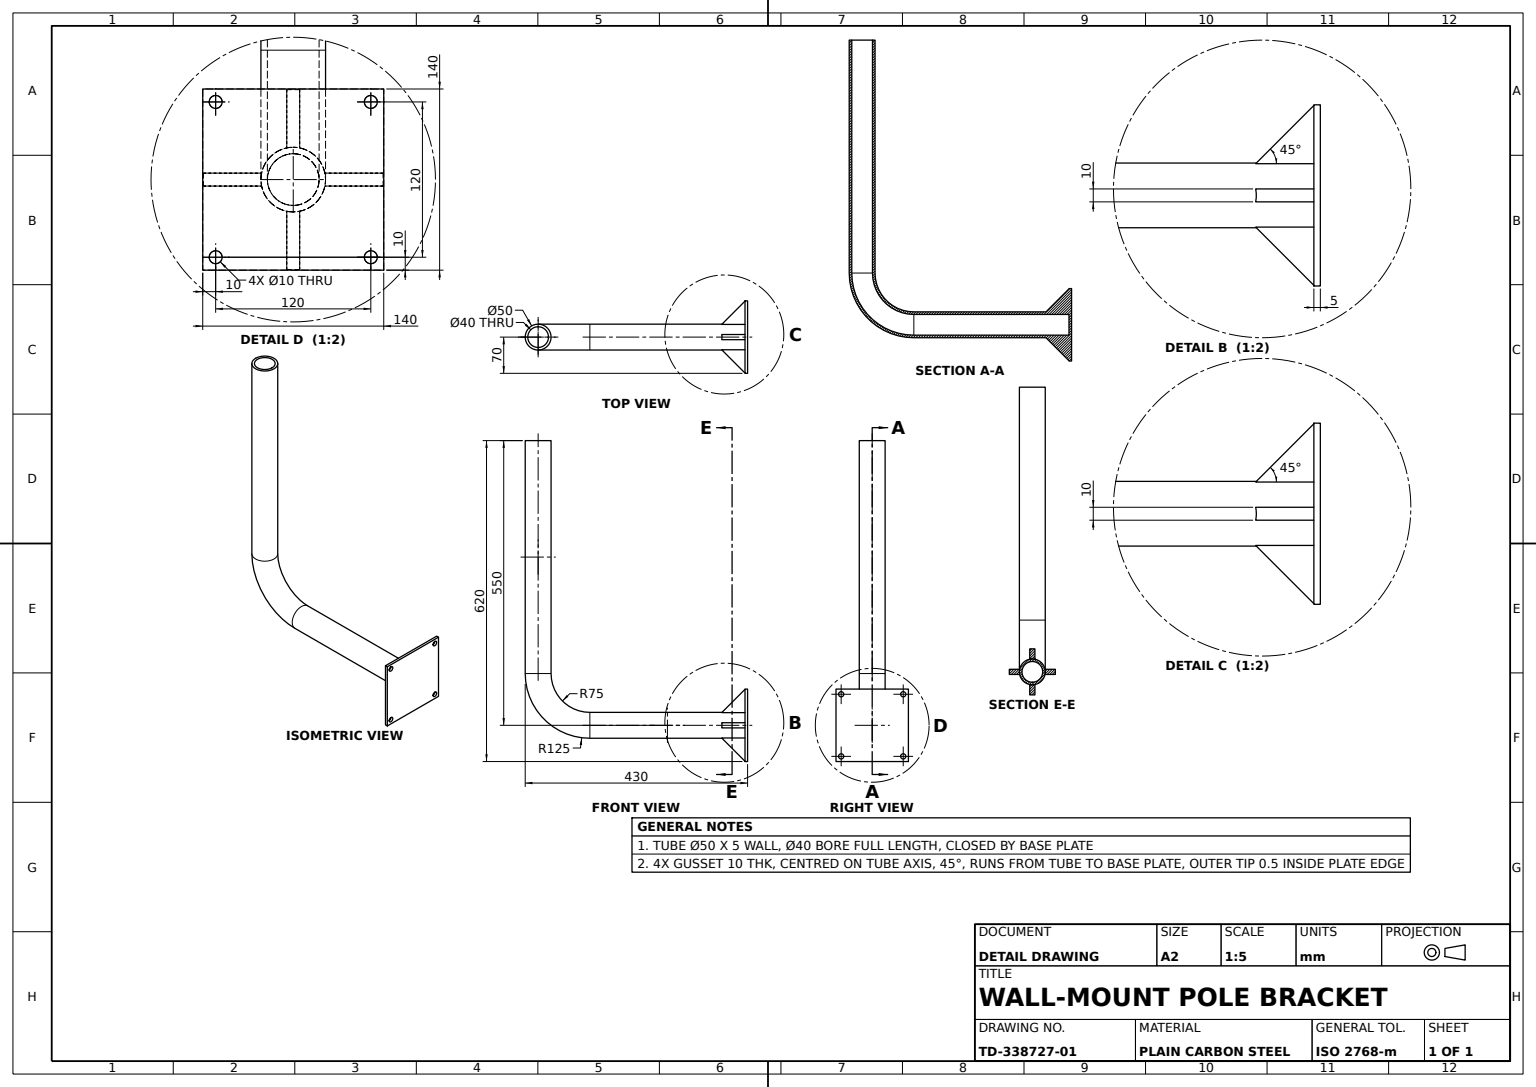
ISO-10303-21;
HEADER;
FILE_DESCRIPTION((''),'2;1');
FILE_NAME('','',(''),(''),'','','');
FILE_SCHEMA(('AUTOMOTIVE_DESIGN'));
ENDSEC;
DATA;
#1=APPLICATION_CONTEXT('');
#2=PRODUCT_CONTEXT('',#1,'mechanical');
#3=PRODUCT('','','',(#2));
#4=PRODUCT_DEFINITION_FORMATION('','',#3);
#5=PRODUCT_DEFINITION_CONTEXT('',#1,'design');
#6=PRODUCT_DEFINITION('','',#4,#5);
#7=PRODUCT_DEFINITION_SHAPE('','',#6);
#8=(LENGTH_UNIT()NAMED_UNIT(*)SI_UNIT(.MILLI.,.METRE.));
#9=(NAMED_UNIT(*)PLANE_ANGLE_UNIT()SI_UNIT($,.RADIAN.));
#10=(NAMED_UNIT(*)SI_UNIT($,.STERADIAN.)SOLID_ANGLE_UNIT());
#11=UNCERTAINTY_MEASURE_WITH_UNIT(LENGTH_MEASURE(1.E-05),#8,'distance_accuracy_value','');
#12=(GEOMETRIC_REPRESENTATION_CONTEXT(3)GLOBAL_UNCERTAINTY_ASSIGNED_CONTEXT((#11))GLOBAL_UNIT_ASSIGNED_CONTEXT((#8,#9,#10))REPRESENTATION_CONTEXT('',''));
#13=CARTESIAN_POINT('',(-120.,450.,0.));
#14=VERTEX_POINT('',#13);
#15=CARTESIAN_POINT('',(-120.,0.,0.));
#16=VERTEX_POINT('',#15);
#17=DIRECTION('',(0.,-1.,0.));
#18=VECTOR('',#17,1000.);
#19=LINE('',#13,#18);
#20=EDGE_CURVE('',#14,#16,#19,.T.);
#21=ORIENTED_EDGE('',*,*,#20,.F.);
#22=CARTESIAN_POINT('',(-80.,450.,0.));
#23=VERTEX_POINT('',#22);
#24=CARTESIAN_POINT('',(-100.,450.,0.));
#25=DIRECTION('',(0.,1.,0.));
#26=DIRECTION('',(-1.,0.,0.));
#27=AXIS2_PLACEMENT_3D('',#24,#25,#26);
#28=CIRCLE('',#27,20.);
#29=EDGE_CURVE('',#14,#23,#28,.T.);
#30=ORIENTED_EDGE('',*,*,#29,.T.);
#31=CARTESIAN_POINT('',(-80.,0.,0.));
#32=VERTEX_POINT('',#31);
#33=LINE('',#22,#18);
#34=EDGE_CURVE('',#23,#32,#33,.T.);
#35=ORIENTED_EDGE('',*,*,#34,.T.);
#36=CARTESIAN_POINT('',(-100.,0.,0.));
#37=DIRECTION('',(1.,0.,0.));
#38=AXIS2_PLACEMENT_3D('',#36,#25,#37);
#39=CIRCLE('',#38,20.);
#40=EDGE_CURVE('',#16,#32,#39,.T.);
#41=ORIENTED_EDGE('',*,*,#40,.F.);
#42=EDGE_LOOP('',(#21,#30,#35,#41));
#43=FACE_OUTER_BOUND('',#42,.T.);
#44=AXIS2_PLACEMENT_3D('',#24,#17,#37);
#45=CYLINDRICAL_SURFACE('',#44,20.);
#46=ADVANCED_FACE('',(#43),#45,.F.);
#47=CARTESIAN_POINT('',(305.,-40.,-55.));
#48=VERTEX_POINT('',#47);
#49=CARTESIAN_POINT('',(305.,-40.,-65.));
#50=VERTEX_POINT('',#49);
#51=CARTESIAN_POINT('',(305.,-40.,-60.));
#52=DIRECTION('',(0.,0.,-1.));
#53=AXIS2_PLACEMENT_3D('',#51,#37,#52);
#54=CIRCLE('',#53,5.);
#55=EDGE_CURVE('',#48,#50,#54,.T.);
#56=ORIENTED_EDGE('',*,*,#55,.T.);
#57=CARTESIAN_POINT('',(300.,-40.,-65.));
#58=VERTEX_POINT('',#57);
#59=CARTESIAN_POINT('',(260.,-40.,-65.));
#60=VECTOR('',#37,1000.);
#61=LINE('',#59,#60);
#62=EDGE_CURVE('',#58,#50,#61,.T.);
#63=ORIENTED_EDGE('',*,*,#62,.F.);
#64=CARTESIAN_POINT('',(300.,-40.,-55.));
#65=VERTEX_POINT('',#64);
#66=CARTESIAN_POINT('',(300.,-40.,-60.));
#67=AXIS2_PLACEMENT_3D('',#66,#37,#52);
#68=CIRCLE('',#67,5.);
#69=EDGE_CURVE('',#65,#58,#68,.T.);
#70=ORIENTED_EDGE('',*,*,#69,.F.);
#71=CARTESIAN_POINT('',(260.,-40.,-55.));
#72=LINE('',#71,#60);
#73=EDGE_CURVE('',#65,#48,#72,.T.);
#74=ORIENTED_EDGE('',*,*,#73,.T.);
#75=EDGE_LOOP('',(#56,#63,#70,#74));
#76=FACE_OUTER_BOUND('',#75,.T.);
#77=CARTESIAN_POINT('',(260.,-40.,-60.));
#78=AXIS2_PLACEMENT_3D('',#77,#37,#52);
#79=CYLINDRICAL_SURFACE('',#78,5.);
#80=ADVANCED_FACE('',(#76),#79,.F.);
#81=CARTESIAN_POINT('',(0.,-125.,0.));
#82=VERTEX_POINT('',#81);
#83=CARTESIAN_POINT('',(255.5,-125.,0.));
#84=VERTEX_POINT('',#83);
#85=LINE('',#81,#60);
#86=EDGE_CURVE('',#82,#84,#85,.T.);
#87=ORIENTED_EDGE('',*,*,#86,.F.);
#88=CARTESIAN_POINT('',(0.,-75.,0.));
#89=VERTEX_POINT('',#88);
#90=CARTESIAN_POINT('',(0.,-100.,0.));
#91=DIRECTION('',(0.,0.,1.));
#92=AXIS2_PLACEMENT_3D('',#90,#26,#91);
#93=CIRCLE('',#92,25.);
#94=EDGE_CURVE('',#89,#82,#93,.T.);
#95=ORIENTED_EDGE('',*,*,#94,.F.);
#96=CARTESIAN_POINT('',(255.5,-75.,0.));
#97=VERTEX_POINT('',#96);
#98=LINE('',#88,#60);
#99=EDGE_CURVE('',#89,#97,#98,.T.);
#100=ORIENTED_EDGE('',*,*,#99,.T.);
#101=CARTESIAN_POINT('',(254.994897,-75.505103,-5.));
#102=VERTEX_POINT('',#101);
#103=CARTESIAN_POINT('',(255.5,-75.,-1.680824));
#104=CARTESIAN_POINT('',(255.331062,-75.168938,-3.353136));
#105=(BOUNDED_CURVE()B_SPLINE_CURVE(3,(#96,#103,#104,#101),.UNSPECIFIED.,.F.,.F.)B_SPLINE_CURVE_WITH_KNOTS((4,4),(0.,0.201357921),.UNSPECIFIED.)CURVE()GEOMETRIC_REPRESENTATION_ITEM()RATIONAL_B_SPLINE_CURVE((1.,0.996624102,0.996624102,1.))REPRESENTATION_ITEM(''));
#106=EDGE_CURVE('',#97,#102,#105,.T.);
#107=ORIENTED_EDGE('',*,*,#106,.T.);
#108=CARTESIAN_POINT('',(300.,-75.505103,-5.));
#109=VERTEX_POINT('',#108);
#110=CARTESIAN_POINT('',(0.,-75.505103,-5.));
#111=VECTOR('',#26,1000.);
#112=LINE('',#110,#111);
#113=EDGE_CURVE('',#109,#102,#112,.T.);
#114=ORIENTED_EDGE('',*,*,#113,.F.);
#115=CARTESIAN_POINT('',(300.,-95.,-24.494897));
#116=VERTEX_POINT('',#115);
#117=CARTESIAN_POINT('',(300.,-100.,0.));
#118=AXIS2_PLACEMENT_3D('',#117,#37,#52);
#119=CIRCLE('',#118,25.);
#120=EDGE_CURVE('',#116,#109,#119,.T.);
#121=ORIENTED_EDGE('',*,*,#120,.F.);
#122=CARTESIAN_POINT('',(254.994897,-95.,-24.494897));
#123=VERTEX_POINT('',#122);
#124=CARTESIAN_POINT('',(0.,-95.,-24.494897));
#125=LINE('',#124,#60);
#126=EDGE_CURVE('',#123,#116,#125,.T.);
#127=ORIENTED_EDGE('',*,*,#126,.F.);
#128=CARTESIAN_POINT('',(254.994897,-105.,-24.494897));
#129=VERTEX_POINT('',#128);
#130=CARTESIAN_POINT('',(255.670666,-98.310578,-25.170666));
#131=CARTESIAN_POINT('',(255.670666,-101.689422,-25.170666));
#132=(BOUNDED_CURVE()B_SPLINE_CURVE(3,(#122,#130,#131,#128),.UNSPECIFIED.,.F.,.F.)B_SPLINE_CURVE_WITH_KNOTS((4,4),(6.081827386,6.484543228),.UNSPECIFIED.)CURVE()GEOMETRIC_REPRESENTATION_ITEM()RATIONAL_B_SPLINE_CURVE((1.,0.986530598,0.986530598,1.))REPRESENTATION_ITEM(''));
#133=EDGE_CURVE('',#123,#129,#132,.T.);
#134=ORIENTED_EDGE('',*,*,#133,.T.);
#135=CARTESIAN_POINT('',(300.,-105.,-24.494897));
#136=VERTEX_POINT('',#135);
#137=CARTESIAN_POINT('',(0.,-105.,-24.494897));
#138=LINE('',#137,#60);
#139=EDGE_CURVE('',#129,#136,#138,.T.);
#140=ORIENTED_EDGE('',*,*,#139,.T.);
#141=CARTESIAN_POINT('',(300.,-124.494897,-5.));
#142=VERTEX_POINT('',#141);
#143=EDGE_CURVE('',#142,#136,#119,.T.);
#144=ORIENTED_EDGE('',*,*,#143,.F.);
#145=CARTESIAN_POINT('',(254.994897,-124.494897,-5.));
#146=VERTEX_POINT('',#145);
#147=CARTESIAN_POINT('',(0.,-124.494897,-5.));
#148=LINE('',#147,#60);
#149=EDGE_CURVE('',#146,#142,#148,.T.);
#150=ORIENTED_EDGE('',*,*,#149,.F.);
#151=CARTESIAN_POINT('',(255.331062,-124.831062,-3.353136));
#152=CARTESIAN_POINT('',(255.5,-125.,-1.680824));
#153=(BOUNDED_CURVE()B_SPLINE_CURVE(3,(#145,#151,#152,#83),.UNSPECIFIED.,.F.,.F.)B_SPLINE_CURVE_WITH_KNOTS((4,4),(6.081827386,6.283185307),.UNSPECIFIED.)CURVE()GEOMETRIC_REPRESENTATION_ITEM()RATIONAL_B_SPLINE_CURVE((1.,0.996624102,0.996624102,1.))REPRESENTATION_ITEM(''));
#154=EDGE_CURVE('',#146,#84,#153,.T.);
#155=ORIENTED_EDGE('',*,*,#154,.T.);
#156=EDGE_LOOP('',(#87,#95,#100,#107,#114,#121,#127,#134,#140,#144,#150,#155));
#157=FACE_OUTER_BOUND('',#156,.T.);
#158=AXIS2_PLACEMENT_3D('',#90,#37,#25);
#159=CYLINDRICAL_SURFACE('',#158,25.);
#160=ADVANCED_FACE('',(#157),#159,.T.);
#161=CARTESIAN_POINT('',(305.,-160.,-65.));
#162=VERTEX_POINT('',#161);
#163=CARTESIAN_POINT('',(305.,-160.,-55.));
#164=VERTEX_POINT('',#163);
#165=CARTESIAN_POINT('',(305.,-160.,-60.));
#166=AXIS2_PLACEMENT_3D('',#165,#37,#52);
#167=CIRCLE('',#166,5.);
#168=EDGE_CURVE('',#162,#164,#167,.T.);
#169=ORIENTED_EDGE('',*,*,#168,.T.);
#170=CARTESIAN_POINT('',(300.,-160.,-55.));
#171=VERTEX_POINT('',#170);
#172=CARTESIAN_POINT('',(260.,-160.,-55.));
#173=LINE('',#172,#60);
#174=EDGE_CURVE('',#171,#164,#173,.T.);
#175=ORIENTED_EDGE('',*,*,#174,.F.);
#176=CARTESIAN_POINT('',(300.,-160.,-65.));
#177=VERTEX_POINT('',#176);
#178=CARTESIAN_POINT('',(300.,-160.,-60.));
#179=AXIS2_PLACEMENT_3D('',#178,#37,#52);
#180=CIRCLE('',#179,5.);
#181=EDGE_CURVE('',#177,#171,#180,.T.);
#182=ORIENTED_EDGE('',*,*,#181,.F.);
#183=CARTESIAN_POINT('',(260.,-160.,-65.));
#184=LINE('',#183,#60);
#185=EDGE_CURVE('',#177,#162,#184,.T.);
#186=ORIENTED_EDGE('',*,*,#185,.T.);
#187=EDGE_LOOP('',(#169,#175,#182,#186));
#188=FACE_OUTER_BOUND('',#187,.T.);
#189=CARTESIAN_POINT('',(260.,-160.,-60.));
#190=AXIS2_PLACEMENT_3D('',#189,#37,#52);
#191=CYLINDRICAL_SURFACE('',#190,5.);
#192=ADVANCED_FACE('',(#188),#191,.F.);
#193=CARTESIAN_POINT('',(300.,-160.,65.));
#194=VERTEX_POINT('',#193);
#195=CARTESIAN_POINT('',(305.,-160.,65.));
#196=VERTEX_POINT('',#195);
#197=CARTESIAN_POINT('',(260.,-160.,65.));
#198=LINE('',#197,#60);
#199=EDGE_CURVE('',#194,#196,#198,.T.);
#200=ORIENTED_EDGE('',*,*,#199,.T.);
#201=CARTESIAN_POINT('',(305.,-160.,55.));
#202=VERTEX_POINT('',#201);
#203=CARTESIAN_POINT('',(305.,-160.,60.));
#204=AXIS2_PLACEMENT_3D('',#203,#37,#52);
#205=CIRCLE('',#204,5.);
#206=EDGE_CURVE('',#196,#202,#205,.T.);
#207=ORIENTED_EDGE('',*,*,#206,.T.);
#208=CARTESIAN_POINT('',(300.,-160.,55.));
#209=VERTEX_POINT('',#208);
#210=CARTESIAN_POINT('',(260.,-160.,55.));
#211=LINE('',#210,#60);
#212=EDGE_CURVE('',#209,#202,#211,.T.);
#213=ORIENTED_EDGE('',*,*,#212,.F.);
#214=CARTESIAN_POINT('',(300.,-160.,60.));
#215=AXIS2_PLACEMENT_3D('',#214,#37,#52);
#216=CIRCLE('',#215,5.);
#217=EDGE_CURVE('',#194,#209,#216,.T.);
#218=ORIENTED_EDGE('',*,*,#217,.F.);
#219=EDGE_LOOP('',(#200,#207,#213,#218));
#220=FACE_OUTER_BOUND('',#219,.T.);
#221=CARTESIAN_POINT('',(260.,-160.,60.));
#222=AXIS2_PLACEMENT_3D('',#221,#37,#52);
#223=CYLINDRICAL_SURFACE('',#222,5.);
#224=ADVANCED_FACE('',(#220),#223,.F.);
#225=EDGE_CURVE('',#58,#65,#68,.T.);
#226=ORIENTED_EDGE('',*,*,#225,.F.);
#227=ORIENTED_EDGE('',*,*,#62,.T.);
#228=EDGE_CURVE('',#50,#48,#54,.T.);
#229=ORIENTED_EDGE('',*,*,#228,.T.);
#230=ORIENTED_EDGE('',*,*,#73,.F.);
#231=EDGE_LOOP('',(#226,#227,#229,#230));
#232=FACE_OUTER_BOUND('',#231,.T.);
#233=ADVANCED_FACE('',(#232),#79,.F.);
#234=CARTESIAN_POINT('',(0.,-120.,0.));
#235=VERTEX_POINT('',#234);
#236=CARTESIAN_POINT('',(0.,0.,0.));
#237=AXIS2_PLACEMENT_3D('',#236,#91,#37);
#238=CIRCLE('',#237,120.);
#239=EDGE_CURVE('',#16,#235,#238,.T.);
#240=ORIENTED_EDGE('',*,*,#239,.F.);
#241=ORIENTED_EDGE('',*,*,#40,.T.);
#242=CARTESIAN_POINT('',(0.,-80.,0.));
#243=VERTEX_POINT('',#242);
#244=CIRCLE('',#237,80.);
#245=EDGE_CURVE('',#32,#243,#244,.T.);
#246=ORIENTED_EDGE('',*,*,#245,.T.);
#247=AXIS2_PLACEMENT_3D('',#90,#26,#17);
#248=CIRCLE('',#247,20.);
#249=EDGE_CURVE('',#235,#243,#248,.T.);
#250=ORIENTED_EDGE('',*,*,#249,.F.);
#251=EDGE_LOOP('',(#240,#241,#246,#250));
#252=FACE_OUTER_BOUND('',#251,.T.);
#253=TOROIDAL_SURFACE('',#237,100.,20.);
#254=ADVANCED_FACE('',(#252),#253,.F.);
#255=EDGE_CURVE('',#243,#235,#248,.T.);
#256=ORIENTED_EDGE('',*,*,#255,.T.);
#257=CARTESIAN_POINT('',(300.,-120.,0.));
#258=VERTEX_POINT('',#257);
#259=LINE('',#234,#60);
#260=EDGE_CURVE('',#235,#258,#259,.T.);
#261=ORIENTED_EDGE('',*,*,#260,.T.);
#262=CARTESIAN_POINT('',(300.,-80.,0.));
#263=VERTEX_POINT('',#262);
#264=CIRCLE('',#118,20.);
#265=EDGE_CURVE('',#258,#263,#264,.T.);
#266=ORIENTED_EDGE('',*,*,#265,.T.);
#267=LINE('',#242,#60);
#268=EDGE_CURVE('',#243,#263,#267,.T.);
#269=ORIENTED_EDGE('',*,*,#268,.F.);
#270=EDGE_LOOP('',(#256,#261,#266,#269));
#271=FACE_OUTER_BOUND('',#270,.T.);
#272=CYLINDRICAL_SURFACE('',#158,20.);
#273=ADVANCED_FACE('',(#271),#272,.F.);
#274=CARTESIAN_POINT('',(-125.,450.,0.));
#275=VERTEX_POINT('',#274);
#276=CARTESIAN_POINT('',(-75.,450.,0.));
#277=VERTEX_POINT('',#276);
#278=AXIS2_PLACEMENT_3D('',#24,#25,#91);
#279=CIRCLE('',#278,25.);
#280=EDGE_CURVE('',#275,#277,#279,.T.);
#281=ORIENTED_EDGE('',*,*,#280,.F.);
#282=CARTESIAN_POINT('',(-125.,0.,0.));
#283=VERTEX_POINT('',#282);
#284=LINE('',#274,#18);
#285=EDGE_CURVE('',#275,#283,#284,.T.);
#286=ORIENTED_EDGE('',*,*,#285,.T.);
#287=CARTESIAN_POINT('',(-75.,0.,0.));
#288=VERTEX_POINT('',#287);
#289=AXIS2_PLACEMENT_3D('',#36,#25,#91);
#290=CIRCLE('',#289,25.);
#291=EDGE_CURVE('',#283,#288,#290,.T.);
#292=ORIENTED_EDGE('',*,*,#291,.T.);
#293=LINE('',#276,#18);
#294=EDGE_CURVE('',#277,#288,#293,.T.);
#295=ORIENTED_EDGE('',*,*,#294,.F.);
#296=EDGE_LOOP('',(#281,#286,#292,#295));
#297=FACE_OUTER_BOUND('',#296,.T.);
#298=CYLINDRICAL_SURFACE('',#44,25.);
#299=ADVANCED_FACE('',(#297),#298,.T.);
#300=CARTESIAN_POINT('',(300.,-30.,70.));
#301=VERTEX_POINT('',#300);
#302=CARTESIAN_POINT('',(305.,-30.,70.));
#303=VERTEX_POINT('',#302);
#304=LINE('',#300,#60);
#305=EDGE_CURVE('',#301,#303,#304,.T.);
#306=ORIENTED_EDGE('',*,*,#305,.T.);
#307=CARTESIAN_POINT('',(305.,-30.,-70.));
#308=VERTEX_POINT('',#307);
#309=VECTOR('',#91,1000.);
#310=LINE('',#302,#309);
#311=EDGE_CURVE('',#308,#303,#310,.T.);
#312=ORIENTED_EDGE('',*,*,#311,.F.);
#313=CARTESIAN_POINT('',(300.,-30.,-70.));
#314=VERTEX_POINT('',#313);
#315=LINE('',#313,#60);
#316=EDGE_CURVE('',#314,#308,#315,.T.);
#317=ORIENTED_EDGE('',*,*,#316,.F.);
#318=LINE('',#300,#309);
#319=EDGE_CURVE('',#314,#301,#318,.T.);
#320=ORIENTED_EDGE('',*,*,#319,.T.);
#321=EDGE_LOOP('',(#306,#312,#317,#320));
#322=FACE_OUTER_BOUND('',#321,.T.);
#323=AXIS2_PLACEMENT_3D('',#300,#25,#91);
#324=PLANE('',#323);
#325=ADVANCED_FACE('',(#322),#324,.T.);
#326=ORIENTED_EDGE('',*,*,#55,.F.);
#327=ORIENTED_EDGE('',*,*,#228,.F.);
#328=EDGE_LOOP('',(#326,#327));
#329=FACE_BOUND('',#328,.T.);
#330=EDGE_CURVE('',#164,#162,#167,.T.);
#331=ORIENTED_EDGE('',*,*,#330,.F.);
#332=ORIENTED_EDGE('',*,*,#168,.F.);
#333=EDGE_LOOP('',(#331,#332));
#334=FACE_BOUND('',#333,.T.);
#335=CARTESIAN_POINT('',(305.,-170.,70.));
#336=VERTEX_POINT('',#335);
#337=LINE('',#302,#18);
#338=EDGE_CURVE('',#303,#336,#337,.T.);
#339=ORIENTED_EDGE('',*,*,#338,.T.);
#340=CARTESIAN_POINT('',(305.,-170.,-70.));
#341=VERTEX_POINT('',#340);
#342=VECTOR('',#52,1000.);
#343=LINE('',#335,#342);
#344=EDGE_CURVE('',#336,#341,#343,.T.);
#345=ORIENTED_EDGE('',*,*,#344,.T.);
#346=VECTOR('',#25,1000.);
#347=LINE('',#307,#346);
#348=EDGE_CURVE('',#341,#308,#347,.T.);
#349=ORIENTED_EDGE('',*,*,#348,.T.);
#350=ORIENTED_EDGE('',*,*,#311,.T.);
#351=EDGE_LOOP('',(#339,#345,#349,#350));
#352=FACE_OUTER_BOUND('',#351,.T.);
#353=CARTESIAN_POINT('',(305.,-40.,55.));
#354=VERTEX_POINT('',#353);
#355=CARTESIAN_POINT('',(305.,-40.,65.));
#356=VERTEX_POINT('',#355);
#357=CARTESIAN_POINT('',(305.,-40.,60.));
#358=AXIS2_PLACEMENT_3D('',#357,#37,#52);
#359=CIRCLE('',#358,5.);
#360=EDGE_CURVE('',#354,#356,#359,.T.);
#361=ORIENTED_EDGE('',*,*,#360,.F.);
#362=EDGE_CURVE('',#356,#354,#359,.T.);
#363=ORIENTED_EDGE('',*,*,#362,.F.);
#364=EDGE_LOOP('',(#361,#363));
#365=FACE_BOUND('',#364,.T.);
#366=ORIENTED_EDGE('',*,*,#206,.F.);
#367=EDGE_CURVE('',#202,#196,#205,.T.);
#368=ORIENTED_EDGE('',*,*,#367,.F.);
#369=EDGE_LOOP('',(#366,#368));
#370=FACE_BOUND('',#369,.T.);
#371=CARTESIAN_POINT('',(305.,-100.,0.));
#372=AXIS2_PLACEMENT_3D('',#371,#26,#91);
#373=PLANE('',#372);
#374=ADVANCED_FACE('',(#329,#334,#352,#365,#370),#373,.F.);
#375=ORIENTED_EDGE('',*,*,#316,.T.);
#376=ORIENTED_EDGE('',*,*,#348,.F.);
#377=CARTESIAN_POINT('',(300.,-170.,-70.));
#378=VERTEX_POINT('',#377);
#379=LINE('',#377,#60);
#380=EDGE_CURVE('',#378,#341,#379,.T.);
#381=ORIENTED_EDGE('',*,*,#380,.F.);
#382=LINE('',#313,#346);
#383=EDGE_CURVE('',#378,#314,#382,.T.);
#384=ORIENTED_EDGE('',*,*,#383,.T.);
#385=EDGE_LOOP('',(#375,#376,#381,#384));
#386=FACE_OUTER_BOUND('',#385,.T.);
#387=AXIS2_PLACEMENT_3D('',#313,#52,#25);
#388=PLANE('',#387);
#389=ADVANCED_FACE('',(#386),#388,.T.);
#390=CARTESIAN_POINT('',(300.,-40.,55.));
#391=VERTEX_POINT('',#390);
#392=CARTESIAN_POINT('',(260.,-40.,55.));
#393=LINE('',#392,#60);
#394=EDGE_CURVE('',#391,#354,#393,.T.);
#395=ORIENTED_EDGE('',*,*,#394,.F.);
#396=CARTESIAN_POINT('',(300.,-40.,65.));
#397=VERTEX_POINT('',#396);
#398=CARTESIAN_POINT('',(300.,-40.,60.));
#399=AXIS2_PLACEMENT_3D('',#398,#37,#52);
#400=CIRCLE('',#399,5.);
#401=EDGE_CURVE('',#397,#391,#400,.T.);
#402=ORIENTED_EDGE('',*,*,#401,.F.);
#403=CARTESIAN_POINT('',(260.,-40.,65.));
#404=LINE('',#403,#60);
#405=EDGE_CURVE('',#397,#356,#404,.T.);
#406=ORIENTED_EDGE('',*,*,#405,.T.);
#407=ORIENTED_EDGE('',*,*,#362,.T.);
#408=EDGE_LOOP('',(#395,#402,#406,#407));
#409=FACE_OUTER_BOUND('',#408,.T.);
#410=CARTESIAN_POINT('',(260.,-40.,60.));
#411=AXIS2_PLACEMENT_3D('',#410,#37,#52);
#412=CYLINDRICAL_SURFACE('',#411,5.);
#413=ADVANCED_FACE('',(#409),#412,.F.);
#414=ORIENTED_EDGE('',*,*,#113,.T.);
#415=CARTESIAN_POINT('',(300.,-30.5,-5.));
#416=VERTEX_POINT('',#415);
#417=CARTESIAN_POINT('',(255.5,-75.,-5.));
#418=DIRECTION('',(0.707106781,0.707106781,0.));
#419=VECTOR('',#418,1000.);
#420=LINE('',#417,#419);
#421=EDGE_CURVE('',#102,#416,#420,.T.);
#422=ORIENTED_EDGE('',*,*,#421,.T.);
#423=CARTESIAN_POINT('',(300.,0.,-5.));
#424=LINE('',#423,#18);
#425=EDGE_CURVE('',#416,#109,#424,.T.);
#426=ORIENTED_EDGE('',*,*,#425,.T.);
#427=EDGE_LOOP('',(#414,#422,#426));
#428=FACE_OUTER_BOUND('',#427,.T.);
#429=CARTESIAN_POINT('',(90.,140.,-5.));
#430=AXIS2_PLACEMENT_3D('',#429,#91,#37);
#431=PLANE('',#430);
#432=ADVANCED_FACE('',(#428),#431,.F.);
#433=CARTESIAN_POINT('',(254.994897,-75.505103,5.));
#434=VERTEX_POINT('',#433);
#435=CARTESIAN_POINT('',(255.331062,-75.168938,3.353136));
#436=CARTESIAN_POINT('',(255.5,-75.,1.680824));
#437=(BOUNDED_CURVE()B_SPLINE_CURVE(3,(#433,#435,#436,#96),.UNSPECIFIED.,.F.,.F.)B_SPLINE_CURVE_WITH_KNOTS((4,4),(6.081827386,6.283185307),.UNSPECIFIED.)CURVE()GEOMETRIC_REPRESENTATION_ITEM()RATIONAL_B_SPLINE_CURVE((1.,0.996624102,0.996624102,1.))REPRESENTATION_ITEM(''));
#438=EDGE_CURVE('',#434,#97,#437,.T.);
#439=ORIENTED_EDGE('',*,*,#438,.F.);
#440=CARTESIAN_POINT('',(300.,-30.5,5.));
#441=VERTEX_POINT('',#440);
#442=CARTESIAN_POINT('',(255.5,-75.,5.));
#443=LINE('',#442,#419);
#444=EDGE_CURVE('',#434,#441,#443,.T.);
#445=ORIENTED_EDGE('',*,*,#444,.T.);
#446=CARTESIAN_POINT('',(300.,-30.5,0.));
#447=LINE('',#446,#309);
#448=EDGE_CURVE('',#416,#441,#447,.T.);
#449=ORIENTED_EDGE('',*,*,#448,.F.);
#450=ORIENTED_EDGE('',*,*,#421,.F.);
#451=ORIENTED_EDGE('',*,*,#106,.F.);
#452=EDGE_LOOP('',(#439,#445,#449,#450,#451));
#453=FACE_OUTER_BOUND('',#452,.T.);
#454=DIRECTION('',(0.707106781,-0.707106781,0.));
#455=AXIS2_PLACEMENT_3D('',#96,#454,#418);
#456=PLANE('',#455);
#457=ADVANCED_FACE('',(#453),#456,.F.);
#458=EDGE_CURVE('',#82,#89,#93,.T.);
#459=ORIENTED_EDGE('',*,*,#458,.T.);
#460=CIRCLE('',#237,75.);
#461=EDGE_CURVE('',#288,#89,#460,.T.);
#462=ORIENTED_EDGE('',*,*,#461,.F.);
#463=ORIENTED_EDGE('',*,*,#291,.F.);
#464=CIRCLE('',#237,125.);
#465=EDGE_CURVE('',#283,#82,#464,.T.);
#466=ORIENTED_EDGE('',*,*,#465,.T.);
#467=EDGE_LOOP('',(#459,#462,#463,#466));
#468=FACE_OUTER_BOUND('',#467,.T.);
#469=TOROIDAL_SURFACE('',#237,100.,25.);
#470=ADVANCED_FACE('',(#468),#469,.T.);
#471=CARTESIAN_POINT('',(300.,-105.,-69.5));
#472=VERTEX_POINT('',#471);
#473=CARTESIAN_POINT('',(300.,-105.,0.));
#474=LINE('',#473,#342);
#475=EDGE_CURVE('',#136,#472,#474,.T.);
#476=ORIENTED_EDGE('',*,*,#475,.F.);
#477=ORIENTED_EDGE('',*,*,#139,.F.);
#478=DIRECTION('',(-0.707106781,0.,0.707106781));
#479=VECTOR('',#478,1000.);
#480=LINE('',#471,#479);
#481=EDGE_CURVE('',#472,#129,#480,.T.);
#482=ORIENTED_EDGE('',*,*,#481,.F.);
#483=EDGE_LOOP('',(#476,#477,#482));
#484=FACE_OUTER_BOUND('',#483,.T.);
#485=CARTESIAN_POINT('',(90.,-105.,0.));
#486=AXIS2_PLACEMENT_3D('',#485,#17,#37);
#487=PLANE('',#486);
#488=ADVANCED_FACE('',(#484),#487,.T.);
#489=ORIENTED_EDGE('',*,*,#344,.F.);
#490=CARTESIAN_POINT('',(300.,-170.,70.));
#491=VERTEX_POINT('',#490);
#492=LINE('',#490,#60);
#493=EDGE_CURVE('',#491,#336,#492,.T.);
#494=ORIENTED_EDGE('',*,*,#493,.F.);
#495=LINE('',#490,#342);
#496=EDGE_CURVE('',#491,#378,#495,.T.);
#497=ORIENTED_EDGE('',*,*,#496,.T.);
#498=ORIENTED_EDGE('',*,*,#380,.T.);
#499=EDGE_LOOP('',(#489,#494,#497,#498));
#500=FACE_OUTER_BOUND('',#499,.T.);
#501=AXIS2_PLACEMENT_3D('',#490,#17,#52);
#502=PLANE('',#501);
#503=ADVANCED_FACE('',(#500),#502,.T.);
#504=ORIENTED_EDGE('',*,*,#245,.F.);
#505=EDGE_CURVE('',#32,#16,#39,.T.);
#506=ORIENTED_EDGE('',*,*,#505,.T.);
#507=ORIENTED_EDGE('',*,*,#239,.T.);
#508=ORIENTED_EDGE('',*,*,#255,.F.);
#509=EDGE_LOOP('',(#504,#506,#507,#508));
#510=FACE_OUTER_BOUND('',#509,.T.);
#511=ADVANCED_FACE('',(#510),#253,.F.);
#512=LINE('',#300,#18);
#513=EDGE_CURVE('',#301,#491,#512,.T.);
#514=ORIENTED_EDGE('',*,*,#513,.T.);
#515=ORIENTED_EDGE('',*,*,#493,.T.);
#516=ORIENTED_EDGE('',*,*,#338,.F.);
#517=ORIENTED_EDGE('',*,*,#305,.F.);
#518=EDGE_LOOP('',(#514,#515,#516,#517));
#519=FACE_OUTER_BOUND('',#518,.T.);
#520=AXIS2_PLACEMENT_3D('',#300,#91,#17);
#521=PLANE('',#520);
#522=ADVANCED_FACE('',(#519),#521,.T.);
#523=CARTESIAN_POINT('',(254.994897,-105.,24.494897));
#524=VERTEX_POINT('',#523);
#525=CARTESIAN_POINT('',(254.994897,-95.,24.494897));
#526=VERTEX_POINT('',#525);
#527=CARTESIAN_POINT('',(255.670666,-101.689422,25.170666));
#528=CARTESIAN_POINT('',(255.670666,-98.310578,25.170666));
#529=(BOUNDED_CURVE()B_SPLINE_CURVE(3,(#523,#527,#528,#525),.UNSPECIFIED.,.F.,.F.)B_SPLINE_CURVE_WITH_KNOTS((4,4),(6.081827386,6.484543228),.UNSPECIFIED.)CURVE()GEOMETRIC_REPRESENTATION_ITEM()RATIONAL_B_SPLINE_CURVE((1.,0.986530598,0.986530598,1.))REPRESENTATION_ITEM(''));
#530=EDGE_CURVE('',#524,#526,#529,.T.);
#531=ORIENTED_EDGE('',*,*,#530,.F.);
#532=CARTESIAN_POINT('',(300.,-105.,69.5));
#533=VERTEX_POINT('',#532);
#534=DIRECTION('',(0.707106781,0.,0.707106781));
#535=VECTOR('',#534,1000.);
#536=LINE('',#532,#535);
#537=EDGE_CURVE('',#524,#533,#536,.T.);
#538=ORIENTED_EDGE('',*,*,#537,.T.);
#539=CARTESIAN_POINT('',(300.,-95.,69.5));
#540=VERTEX_POINT('',#539);
#541=CARTESIAN_POINT('',(300.,-100.,69.5));
#542=LINE('',#541,#18);
#543=EDGE_CURVE('',#540,#533,#542,.T.);
#544=ORIENTED_EDGE('',*,*,#543,.F.);
#545=LINE('',#539,#535);
#546=EDGE_CURVE('',#526,#540,#545,.T.);
#547=ORIENTED_EDGE('',*,*,#546,.F.);
#548=EDGE_LOOP('',(#531,#538,#544,#547));
#549=FACE_OUTER_BOUND('',#548,.T.);
#550=DIRECTION('',(0.707106781,0.,-0.707106781));
#551=AXIS2_PLACEMENT_3D('',#541,#550,#534);
#552=PLANE('',#551);
#553=ADVANCED_FACE('',(#549),#552,.F.);
#554=ORIENTED_EDGE('',*,*,#199,.F.);
#555=EDGE_CURVE('',#209,#194,#216,.T.);
#556=ORIENTED_EDGE('',*,*,#555,.F.);
#557=ORIENTED_EDGE('',*,*,#212,.T.);
#558=ORIENTED_EDGE('',*,*,#367,.T.);
#559=EDGE_LOOP('',(#554,#556,#557,#558));
#560=FACE_OUTER_BOUND('',#559,.T.);
#561=ADVANCED_FACE('',(#560),#223,.F.);
#562=CARTESIAN_POINT('',(300.,-95.,-69.5));
#563=VERTEX_POINT('',#562);
#564=LINE('',#562,#479);
#565=EDGE_CURVE('',#563,#123,#564,.T.);
#566=ORIENTED_EDGE('',*,*,#565,.F.);
#567=CARTESIAN_POINT('',(300.,-100.,-69.5));
#568=LINE('',#567,#18);
#569=EDGE_CURVE('',#563,#472,#568,.T.);
#570=ORIENTED_EDGE('',*,*,#569,.T.);
#571=ORIENTED_EDGE('',*,*,#481,.T.);
#572=ORIENTED_EDGE('',*,*,#133,.F.);
#573=EDGE_LOOP('',(#566,#570,#571,#572));
#574=FACE_OUTER_BOUND('',#573,.T.);
#575=AXIS2_PLACEMENT_3D('',#567,#534,#478);
#576=PLANE('',#575);
#577=ADVANCED_FACE('',(#574),#576,.F.);
#578=ORIENTED_EDGE('',*,*,#401,.T.);
#579=EDGE_CURVE('',#391,#397,#400,.T.);
#580=ORIENTED_EDGE('',*,*,#579,.T.);
#581=EDGE_LOOP('',(#578,#580));
#582=FACE_BOUND('',#581,.T.);
#583=EDGE_CURVE('',#171,#177,#180,.T.);
#584=ORIENTED_EDGE('',*,*,#583,.T.);
#585=ORIENTED_EDGE('',*,*,#181,.T.);
#586=EDGE_LOOP('',(#584,#585));
#587=FACE_BOUND('',#586,.T.);
#588=CARTESIAN_POINT('',(300.,-169.5,-5.));
#589=VERTEX_POINT('',#588);
#590=CARTESIAN_POINT('',(300.,-169.5,5.));
#591=VERTEX_POINT('',#590);
#592=CARTESIAN_POINT('',(300.,-169.5,0.));
#593=LINE('',#592,#309);
#594=EDGE_CURVE('',#589,#591,#593,.T.);
#595=ORIENTED_EDGE('',*,*,#594,.F.);
#596=EDGE_CURVE('',#142,#589,#424,.T.);
#597=ORIENTED_EDGE('',*,*,#596,.F.);
#598=ORIENTED_EDGE('',*,*,#143,.T.);
#599=ORIENTED_EDGE('',*,*,#475,.T.);
#600=ORIENTED_EDGE('',*,*,#569,.F.);
#601=CARTESIAN_POINT('',(300.,-95.,0.));
#602=LINE('',#601,#342);
#603=EDGE_CURVE('',#116,#563,#602,.T.);
#604=ORIENTED_EDGE('',*,*,#603,.F.);
#605=ORIENTED_EDGE('',*,*,#120,.T.);
#606=ORIENTED_EDGE('',*,*,#425,.F.);
#607=ORIENTED_EDGE('',*,*,#448,.T.);
#608=CARTESIAN_POINT('',(300.,-75.505103,5.));
#609=VERTEX_POINT('',#608);
#610=CARTESIAN_POINT('',(300.,0.,5.));
#611=LINE('',#610,#18);
#612=EDGE_CURVE('',#441,#609,#611,.T.);
#613=ORIENTED_EDGE('',*,*,#612,.T.);
#614=CARTESIAN_POINT('',(300.,-95.,24.494897));
#615=VERTEX_POINT('',#614);
#616=EDGE_CURVE('',#609,#615,#119,.T.);
#617=ORIENTED_EDGE('',*,*,#616,.T.);
#618=EDGE_CURVE('',#540,#615,#602,.T.);
#619=ORIENTED_EDGE('',*,*,#618,.F.);
#620=ORIENTED_EDGE('',*,*,#543,.T.);
#621=CARTESIAN_POINT('',(300.,-105.,24.494897));
#622=VERTEX_POINT('',#621);
#623=EDGE_CURVE('',#533,#622,#474,.T.);
#624=ORIENTED_EDGE('',*,*,#623,.T.);
#625=CARTESIAN_POINT('',(300.,-124.494897,5.));
#626=VERTEX_POINT('',#625);
#627=EDGE_CURVE('',#622,#626,#119,.T.);
#628=ORIENTED_EDGE('',*,*,#627,.T.);
#629=EDGE_CURVE('',#626,#591,#611,.T.);
#630=ORIENTED_EDGE('',*,*,#629,.T.);
#631=EDGE_LOOP('',(#595,#597,#598,#599,#600,#604,#605,#606,#607,#613,#617,#619,#620,#624,#628,#630));
#632=FACE_BOUND('',#631,.T.);
#633=ORIENTED_EDGE('',*,*,#225,.T.);
#634=ORIENTED_EDGE('',*,*,#69,.T.);
#635=EDGE_LOOP('',(#633,#634));
#636=FACE_BOUND('',#635,.T.);
#637=ORIENTED_EDGE('',*,*,#319,.F.);
#638=ORIENTED_EDGE('',*,*,#383,.F.);
#639=ORIENTED_EDGE('',*,*,#496,.F.);
#640=ORIENTED_EDGE('',*,*,#513,.F.);
#641=EDGE_LOOP('',(#637,#638,#639,#640));
#642=FACE_OUTER_BOUND('',#641,.T.);
#643=ORIENTED_EDGE('',*,*,#555,.T.);
#644=ORIENTED_EDGE('',*,*,#217,.T.);
#645=EDGE_LOOP('',(#643,#644));
#646=FACE_BOUND('',#645,.T.);
#647=CARTESIAN_POINT('',(300.,0.,0.));
#648=AXIS2_PLACEMENT_3D('',#647,#37,#52);
#649=PLANE('',#648);
#650=ADVANCED_FACE('',(#582,#587,#632,#636,#642,#646),#649,.F.);
#651=EDGE_CURVE('',#23,#14,#28,.T.);
#652=ORIENTED_EDGE('',*,*,#651,.F.);
#653=ORIENTED_EDGE('',*,*,#29,.F.);
#654=EDGE_LOOP('',(#652,#653));
#655=FACE_BOUND('',#654,.T.);
#656=EDGE_CURVE('',#277,#275,#279,.T.);
#657=ORIENTED_EDGE('',*,*,#656,.T.);
#658=ORIENTED_EDGE('',*,*,#280,.T.);
#659=EDGE_LOOP('',(#657,#658));
#660=FACE_OUTER_BOUND('',#659,.T.);
#661=PLANE('',#278);
#662=ADVANCED_FACE('',(#655,#660),#661,.T.);
#663=CARTESIAN_POINT('',(254.994897,-124.494897,5.));
#664=VERTEX_POINT('',#663);
#665=CARTESIAN_POINT('',(0.,-124.494897,5.));
#666=LINE('',#665,#60);
#667=EDGE_CURVE('',#664,#626,#666,.T.);
#668=ORIENTED_EDGE('',*,*,#667,.F.);
#669=CARTESIAN_POINT('',(255.5,-125.,5.));
#670=VECTOR('',#454,1000.);
#671=LINE('',#669,#670);
#672=EDGE_CURVE('',#664,#591,#671,.T.);
#673=ORIENTED_EDGE('',*,*,#672,.T.);
#674=ORIENTED_EDGE('',*,*,#629,.F.);
#675=EDGE_LOOP('',(#668,#673,#674));
#676=FACE_OUTER_BOUND('',#675,.T.);
#677=CARTESIAN_POINT('',(90.,140.,5.));
#678=AXIS2_PLACEMENT_3D('',#677,#91,#37);
#679=PLANE('',#678);
#680=ADVANCED_FACE('',(#676),#679,.T.);
#681=ORIENTED_EDGE('',*,*,#616,.F.);
#682=CARTESIAN_POINT('',(0.,-75.505103,5.));
#683=LINE('',#682,#111);
#684=EDGE_CURVE('',#609,#434,#683,.T.);
#685=ORIENTED_EDGE('',*,*,#684,.T.);
#686=ORIENTED_EDGE('',*,*,#438,.T.);
#687=ORIENTED_EDGE('',*,*,#99,.F.);
#688=ORIENTED_EDGE('',*,*,#458,.F.);
#689=ORIENTED_EDGE('',*,*,#86,.T.);
#690=CARTESIAN_POINT('',(255.5,-125.,1.680824));
#691=CARTESIAN_POINT('',(255.331062,-124.831062,3.353136));
#692=(BOUNDED_CURVE()B_SPLINE_CURVE(3,(#83,#690,#691,#663),.UNSPECIFIED.,.F.,.T.)B_SPLINE_CURVE_WITH_KNOTS((4,4),(0.,0.201357921),.UNSPECIFIED.)CURVE()GEOMETRIC_REPRESENTATION_ITEM()RATIONAL_B_SPLINE_CURVE((1.,0.996624102,0.996624102,1.))REPRESENTATION_ITEM(''));
#693=EDGE_CURVE('',#84,#664,#692,.T.);
#694=ORIENTED_EDGE('',*,*,#693,.T.);
#695=ORIENTED_EDGE('',*,*,#667,.T.);
#696=ORIENTED_EDGE('',*,*,#627,.F.);
#697=CARTESIAN_POINT('',(0.,-105.,24.494897));
#698=LINE('',#697,#111);
#699=EDGE_CURVE('',#622,#524,#698,.T.);
#700=ORIENTED_EDGE('',*,*,#699,.T.);
#701=ORIENTED_EDGE('',*,*,#530,.T.);
#702=CARTESIAN_POINT('',(0.,-95.,24.494897));
#703=LINE('',#702,#111);
#704=EDGE_CURVE('',#615,#526,#703,.T.);
#705=ORIENTED_EDGE('',*,*,#704,.F.);
#706=EDGE_LOOP('',(#681,#685,#686,#687,#688,#689,#694,#695,#696,#700,#701,#705));
#707=FACE_OUTER_BOUND('',#706,.T.);
#708=ADVANCED_FACE('',(#707),#159,.T.);
#709=ORIENTED_EDGE('',*,*,#594,.T.);
#710=ORIENTED_EDGE('',*,*,#672,.F.);
#711=ORIENTED_EDGE('',*,*,#693,.F.);
#712=ORIENTED_EDGE('',*,*,#154,.F.);
#713=CARTESIAN_POINT('',(255.5,-125.,-5.));
#714=LINE('',#713,#670);
#715=EDGE_CURVE('',#146,#589,#714,.T.);
#716=ORIENTED_EDGE('',*,*,#715,.T.);
#717=EDGE_LOOP('',(#709,#710,#711,#712,#716));
#718=FACE_OUTER_BOUND('',#717,.T.);
#719=DIRECTION('',(-0.707106781,-0.707106781,0.));
#720=AXIS2_PLACEMENT_3D('',#83,#719,#454);
#721=PLANE('',#720);
#722=ADVANCED_FACE('',(#718),#721,.T.);
#723=ORIENTED_EDGE('',*,*,#704,.T.);
#724=ORIENTED_EDGE('',*,*,#546,.T.);
#725=ORIENTED_EDGE('',*,*,#618,.T.);
#726=EDGE_LOOP('',(#723,#724,#725));
#727=FACE_OUTER_BOUND('',#726,.T.);
#728=CARTESIAN_POINT('',(90.,-95.,0.));
#729=AXIS2_PLACEMENT_3D('',#728,#17,#37);
#730=PLANE('',#729);
#731=ADVANCED_FACE('',(#727),#730,.F.);
#732=ORIENTED_EDGE('',*,*,#185,.F.);
#733=ORIENTED_EDGE('',*,*,#583,.F.);
#734=ORIENTED_EDGE('',*,*,#174,.T.);
#735=ORIENTED_EDGE('',*,*,#330,.T.);
#736=EDGE_LOOP('',(#732,#733,#734,#735));
#737=FACE_OUTER_BOUND('',#736,.T.);
#738=ADVANCED_FACE('',(#737),#191,.F.);
#739=EDGE_CURVE('',#263,#258,#264,.T.);
#740=ORIENTED_EDGE('',*,*,#739,.F.);
#741=ORIENTED_EDGE('',*,*,#265,.F.);
#742=EDGE_LOOP('',(#740,#741));
#743=FACE_OUTER_BOUND('',#742,.T.);
#744=ADVANCED_FACE('',(#743),#649,.F.);
#745=ORIENTED_EDGE('',*,*,#715,.F.);
#746=ORIENTED_EDGE('',*,*,#149,.T.);
#747=ORIENTED_EDGE('',*,*,#596,.T.);
#748=EDGE_LOOP('',(#745,#746,#747));
#749=FACE_OUTER_BOUND('',#748,.T.);
#750=ADVANCED_FACE('',(#749),#431,.F.);
#751=ORIENTED_EDGE('',*,*,#461,.T.);
#752=ORIENTED_EDGE('',*,*,#94,.T.);
#753=ORIENTED_EDGE('',*,*,#465,.F.);
#754=EDGE_CURVE('',#288,#283,#290,.T.);
#755=ORIENTED_EDGE('',*,*,#754,.F.);
#756=EDGE_LOOP('',(#751,#752,#753,#755));
#757=FACE_OUTER_BOUND('',#756,.T.);
#758=ADVANCED_FACE('',(#757),#469,.T.);
#759=ORIENTED_EDGE('',*,*,#249,.T.);
#760=ORIENTED_EDGE('',*,*,#268,.T.);
#761=ORIENTED_EDGE('',*,*,#739,.T.);
#762=ORIENTED_EDGE('',*,*,#260,.F.);
#763=EDGE_LOOP('',(#759,#760,#761,#762));
#764=FACE_OUTER_BOUND('',#763,.T.);
#765=ADVANCED_FACE('',(#764),#272,.F.);
#766=ORIENTED_EDGE('',*,*,#623,.F.);
#767=ORIENTED_EDGE('',*,*,#537,.F.);
#768=ORIENTED_EDGE('',*,*,#699,.F.);
#769=EDGE_LOOP('',(#766,#767,#768));
#770=FACE_OUTER_BOUND('',#769,.T.);
#771=ADVANCED_FACE('',(#770),#487,.T.);
#772=ORIENTED_EDGE('',*,*,#285,.F.);
#773=ORIENTED_EDGE('',*,*,#656,.F.);
#774=ORIENTED_EDGE('',*,*,#294,.T.);
#775=ORIENTED_EDGE('',*,*,#754,.T.);
#776=EDGE_LOOP('',(#772,#773,#774,#775));
#777=FACE_OUTER_BOUND('',#776,.T.);
#778=ADVANCED_FACE('',(#777),#298,.T.);
#779=ORIENTED_EDGE('',*,*,#126,.T.);
#780=ORIENTED_EDGE('',*,*,#603,.T.);
#781=ORIENTED_EDGE('',*,*,#565,.T.);
#782=EDGE_LOOP('',(#779,#780,#781));
#783=FACE_OUTER_BOUND('',#782,.T.);
#784=ADVANCED_FACE('',(#783),#730,.F.);
#785=ORIENTED_EDGE('',*,*,#34,.F.);
#786=ORIENTED_EDGE('',*,*,#651,.T.);
#787=ORIENTED_EDGE('',*,*,#20,.T.);
#788=ORIENTED_EDGE('',*,*,#505,.F.);
#789=EDGE_LOOP('',(#785,#786,#787,#788));
#790=FACE_OUTER_BOUND('',#789,.T.);
#791=ADVANCED_FACE('',(#790),#45,.F.);
#792=ORIENTED_EDGE('',*,*,#612,.F.);
#793=ORIENTED_EDGE('',*,*,#444,.F.);
#794=ORIENTED_EDGE('',*,*,#684,.F.);
#795=EDGE_LOOP('',(#792,#793,#794));
#796=FACE_OUTER_BOUND('',#795,.T.);
#797=ADVANCED_FACE('',(#796),#679,.T.);
#798=ORIENTED_EDGE('',*,*,#360,.T.);
#799=ORIENTED_EDGE('',*,*,#405,.F.);
#800=ORIENTED_EDGE('',*,*,#579,.F.);
#801=ORIENTED_EDGE('',*,*,#394,.T.);
#802=EDGE_LOOP('',(#798,#799,#800,#801));
#803=FACE_OUTER_BOUND('',#802,.T.);
#804=ADVANCED_FACE('',(#803),#412,.F.);
#805=CLOSED_SHELL('',(#46,#80,#160,#192,#224,#233,#254,#273,#299,#325,#374,#389,#413,#432,#457,#470,#488,#503,#511,#522,#553,#561,#577,#650,#662,#680,#708,#722,#731,#738,#744,#750,#758,#765,#771,#778,#784,#791,#797,#804));
#806=MANIFOLD_SOLID_BREP('',#805);
#807=ADVANCED_BREP_SHAPE_REPRESENTATION('',(#806),#12);
#808=SHAPE_DEFINITION_REPRESENTATION(#7,#807);
ENDSEC;
END-ISO-10303-21;
